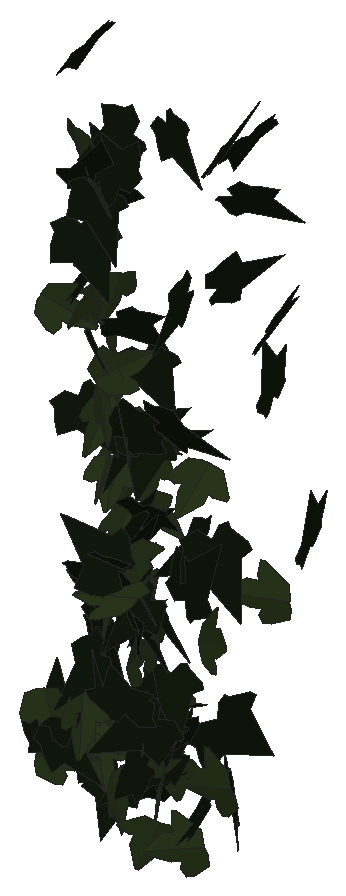
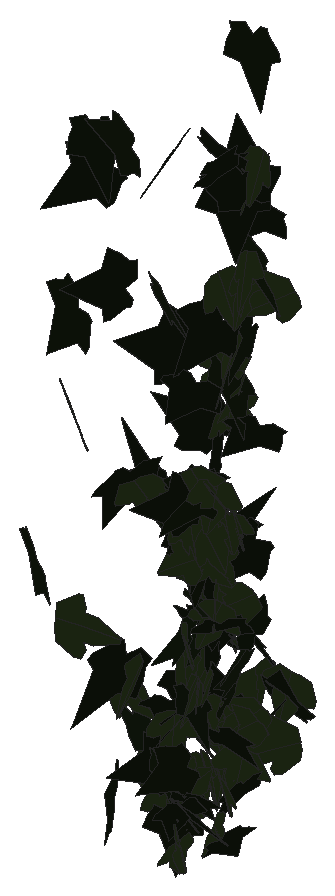
# SketchUp Ruby script. Lengths in inches.
U = 1.inch
M = Sketchup.active_model
def pt(a) = Geom::Point3d.new(a.map { |v| v * U })
def face(e, loops, mat)
  f = e.add_face(loops[0].map { |a| pt(a) })
  loops[1..].each { |l| e.add_face(l.map { |a| pt(a) }).erase! }
  f.material = f.back_material = mat if mat
  f
end
# faces: each face lists its corners as indices into pts; further lists are holes
def faces(e, pts, list, mat = nil) = list.each { |f| face(e, (f[0].is_a?(Array) ? f : [f]).map { |l| l.map { |i| pts[i] } }, mat) }
# xy, xz, yz: faces in a plane at the given z, y or x. An outline is a flat list of corners, or four numbers for a rectangle; further outlines are holes
def ring(l) = l.size == 4 ? [[l[0], l[1]], [l[2], l[1]], [l[2], l[3]], [l[0], l[3]]] : l.each_slice(2).to_a
def flat(e, list, mat, &to3) = list.each { |f| face(e, (f[0].is_a?(Array) ? f : [f]).map { |l| ring(l).map { |u, v| to3.(u, v) } }, mat) }
def xy(e, z, list, mat = nil) = flat(e, list, mat) { |x, y| [x, y, z] }
def xz(e, y, list, mat = nil) = flat(e, list, mat) { |x, z| [x, y, z] }
def yz(e, x, list, mat = nil) = flat(e, list, mat) { |y, z| [x, y, z] }
def lines(e, pts, list) = list.each { |a, b| e.add_line(pt(pts[a]), pt(pts[b])) }
# prism: a flat outline (further loops are holes) pulled along v
def prism(e, loops, v, mat = nil)
  f = face(e, loops, mat); d = Geom::Vector3d.new(v.map { |x| x * U })
  f.pushpull(f.normal.samedirection?(d) ? d.length : -d.length)
end
def box(e, o, s, mat = nil) = prism(e, [[o, [o[0] + s[0], o[1], o[2]], [o[0] + s[0], o[1] + s[1], o[2]], [o[0], o[1] + s[1], o[2]]]], [0, 0, s[2]], mat)
def at(x, y, z, deg = 0) = Geom::Transformation.translation(pt([x, y, z])) * Geom::Transformation.rotation(ORIGIN, Z_AXIS, deg.degrees)
def axes(o, x, y, z) = Geom::Transformation.new([*x, 0, *y, 0, *z, 0, *pt(o).to_a, 1])
def part(name) = M.definitions.add(name)
# library, detail: a bought-in or finely detailed component or shape, given as its bounding box
def library(name, o, s) = part(name).tap { |d| box(d.entities, o, s) }
def detail(e, o, s) = box(e.add_group.entities, o, s)
def put(e, d, t, mat = nil) = e.add_instance(d, t).tap { |i| i.material = mat if mat }
def group(e, t, mat = nil) = e.add_group.tap { |g| g.transformation = t; g.material = mat if mat }.entities
root = M.entities
M.materials.add("efeu1").color = [18, 25, 13]
M.materials.add("efeu2").color = [43, 57, 29]
c1 = part("ivyleaf_9")
p = [[1.54,2.16,1.25],[1.36,2.04,1.19],[-0.21,0.99,0.68],[-0.71,1.11,0.82],[-0.85,0.86,0.67],[-0.8,0.17,0.21],
  [-0.9,-0.01,0.1],[-0.67,-0.16,-0.02],[-0.08,-0.08,-0.05],[-0.03,-0.6,-0.4],[0.65,-0.88,-0.66],[0.83,-0.6,-0.49],
  [1.29,-0.42,-0.43],[1.8125,-0.07,-0.26],[1.21,0.44,0.15]]
faces(c1.entities,p,[[0,1,2,3,4,5,6,7,8,9,10,11,12,13,14]],"efeu1")
c2 = part("ivyleaf_10")
p = [[0,0.5,-0.03],[-0.0625,2.02,-0.43],[-0.19,2.01,-0.46],[-0.54,1.05,-0.29],[-0.52,0.625,-0.18],[-0.83,0.76,-0.28],
  [-1.16,0.64,-0.33],[-1.15,0.33,-0.24],[-0.77,-0.39,0.02],[-0.3,-0.51,0.16],[0.04,-0.48,0.23],[-0.02,2.01,-0.4375],
  [-0.06,2.01,-0.43],[0.04,-0.49,0.23],[0.67,-0.49,0.14],[1.38,0.36,-0.2],[1.375,0.51,-0.24],[0.81,0.65,-0.19],
  [0.62,0.59,-0.15],[0.6,1.09,-0.28],[0.5,1.23,-0.31]]
faces(c2.entities,p,[[0,1,2,3,4,5,6,7,8,9,10],[11,12,0,13,14,15,16,17,18,19,20]],"efeu2")
put(root,c1,axes([599.8,129.43,210.84],[-1.0094,0.32917,0.06825],[0.04265,-0.08885,1.05933],[0.33345,1.0078,0.0711]))
put(root,c2,axes([599.1875,129.7,212.04],[1.03048,0.1413,0.29449],[0.24667,0.30222,-1.00817],[-0.21411,1.02824,0.25585]))
put(root,c1,axes([600.84,130.04,234.19],[-0.38872,-0.56207,-0.84526],[0.63503,0.57147,-0.67204],[0.79191,-0.73416,0.12401]))
put(root,c1,axes([599.62,129.73,210.85],[0.65216,-0.64278,-0.53026],[-0.15877,0.56516,-0.88036],[0.81801,0.62216,0.25187]))
put(root,c2,axes([603.07,129.99,217.9375],[-0.04227,1.23527,0.10042],[-1.23885,-0.04494,0.03131],[0.03483,-0.09925,1.2356]))
put(root,c1,axes([603.22,129.6875,213.04],[-0.18269,1.18347,0.00538],[-1.18301,-0.18277,0.03272],[0.03315,-0.00033,1.19704]))
put(root,c2,axes([600.71,130.22,212.13],[0.2396,0.99661,-0.25674],[-0.03873,-0.25469,-1.02479],[-1.02842,0.24178,-0.02122]))
put(root,c1,axes([601.19,130.41,235.84],[0.22293,-1.02597,-0.19339],[0.03804,0.2056,-1.0469],[1.04335,0.21172,0.07949]))
put(root,c1,axes([606.04,130.19,219.01],[-0.46531,0.47847,0.92349],[0.59746,-0.70516,0.66638],[0.85135,0.75637,0.03708]))
put(root,c2,axes([599.44,129.83,230.4],[0.41584,0.19312,0.89669],[0.64054,0.64358,-0.43565],[-0.65656,0.75019,0.14291]))
put(root,c1,axes([601.23,130.51,214.45],[-1.01027,0.18239,-0.18284],[0.17994,-0.03243,-1.0266],[-0.18525,-1.02617,-0.00006]))
put(root,c1,axes([601.07,130.26,232.3],[-0.69225,0.82547,-0.08837],[0.06963,-0.05693,-1.07718],[-0.82726,-0.69554,-0.01671]))
put(root,c1,axes([601.88,130.83,218.54],[-0.42706,-1.03566,-0.02438],[0.04845,-0.04631,1.11851],[-1.03481,0.42524,0.06243]))
put(root,c1,axes([604.54,130.51,226.29],[0.76824,-0.32958,0.76916],[0.72035,-0.27086,-0.83555],[0.42582,1.05282,0.02582]))
put(root,c2,axes([599.08,130.1,209.22],[0.25287,-0.03046,1.00775],[0.47165,0.92184,-0.09049],[-0.89108,0.47929,0.23808]))
put(root,c2,axes([600.92,130.4375,230.94],[-0.13056,-0.88408,-0.57455],[0.04805,0.57335,-0.89315],[1.05328,-0.13575,-0.03047]))
put(root,c1,axes([600.72,130.33,242.4375],[-0.18071,1.07408,0.03515],[0.00614,0.03667,-1.08911],[-1.07464,-0.18041,-0.01214]))
put(root,c2,axes([600.95,130.64,235.82],[-0.88422,0.59693,0.11629],[-0.09585,0.06585,-1.06685],[-0.60055,-0.8894,-0.00094]))
put(root,c1,axes([600.37,131.18,235.6],[1.00501,0.36415,0.33832],[-0.31892,-0.11293,1.06895],[0.38125,-1.0544,0.00236]))
put(root,c1,axes([603.37,131.51,211.86],[-0.00613,-0.05087,-1.06175],[-0.40107,-0.98318,0.04942],[-0.9844,0.40089,-0.01352]))
put(root,c1,axes([600.66,130.45,218.5625],[0.94908,0.46168,0.16133],[0.12921,0.10297,-1.05482],[-0.47168,0.95718,0.03566]))
put(root,c2,axes([603.59,131.27,206.99],[-0.77742,-0.5951,0.43027],[-0.33296,-0.27283,-0.97896],[0.65453,-0.84562,0.01305]))
put(root,c1,axes([600.53,130.8125,228.82],[0.80974,-0.24262,-0.57743],[-0.55018,0.17548,-0.84527],[0.29931,0.97893,0.00841]))
put(root,c1,axes([602.11,130.7,236.35],[0.0561,0.38948,0.99667],[-0.74296,0.73244,-0.2444],[-0.7701,-0.67826,0.3084]))
put(root,c1,axes([601.125,130.84,235.37],[0.32356,0.9691,-0.29244],[-0.08667,-0.27937,-1.02167],[-1.00854,0.33492,-0.00602]))
put(root,c2,axes([605.35,131.48,206.74],[-0.33312,-0.03273,1.09339],[-1.00318,-0.44656,-0.31901],[0.43613,-1.05217,0.10138]))
put(root,c2,axes([600.78,131.63,225.24],[0.34032,0.79523,-0.57393],[-0.2388,-0.52202,-0.86491],[-0.95119,0.41557,0.0118]))
put(root,c2,axes([607.01,131.3125,210.14],[-0.38104,-0.01996,1.13302],[-1.13181,-0.05252,-0.38156],[0.05614,-1.19423,-0.00215]))
put(root,c2,axes([600.76,131.38,225.91],[-0.26255,0.99795,-0.1218],[0.00806,-0.12379,-1.03164],[-1.00532,-0.26162,0.02354]))
put(root,c2,axes([601.23,131.71,231.13],[-0.33562,-0.94792,0.23589],[-0.08153,-0.22137,-1.00558],[0.97343,-0.34537,-0.00289]))
put(root,c2,axes([599.59,131.36,237.41],[-0.91697,0.40198,0.01413],[-0.01262,0.00641,-1.00121],[-0.40203,-0.91706,-0.0008]))
put(root,c1,axes([605.89,131.68,208.81],[-0.81886,0.74891,-0.2525],[0.1762,-0.18144,-1.10959],[-0.77044,-0.83747,0.0146]))
put(root,c2,axes([601.17,131.21,227.05],[-0.2997,-0.43125,0.90814],[0.46576,0.78024,0.52423],[-0.89094,0.55296,-0.03143]))
put(root,c2,axes([601.32,131.5625,208.09],[-0.24681,0.99933,0.07458],[-0.11536,0.04796,-1.02446],[-0.99545,-0.25333,0.10023]))
put(root,c1,axes([601.14,131.31,226.83],[-0.30172,0.9805,0.14131],[-0.06821,0.1268,-1.0255],[-0.98828,-0.30809,0.02764]))
put(root,c1,axes([602.48,131.95,209.28],[-0.95299,0.34936,-0.02468],[0.01845,-0.02135,-1.01492],[-0.34975,-0.95307,0.01369]))
put(root,c1,axes([599.28,131.8,225.07],[-0.0914,-0.53308,-0.7751],[0.44979,0.6592,-0.50641],[0.82623,-0.41784,0.18994]))
put(root,c2,axes([602.02,132.51,211.35],[0.33567,-0.31147,0.88223],[0.68401,-0.5578,-0.45718],[0.63835,0.76149,0.02597]))
put(root,c1,axes([605.86,132.07,220.625],[0.10017,-1.00887,-0.62351],[-0.07039,0.61957,-1.0138],[1.18391,0.1222,-0.00752]))
put(root,c2,axes([599.81,132.28,209.26],[-0.93136,-0.34751,-0.17806],[0.27999,-0.27337,-0.93101],[0.27216,-0.90797,0.34846]))
put(root,c2,axes([599.78,131.91,232.73],[0.08944,-0.8559,-0.45372],[0.04234,0.45867,-0.85689],[0.9678,0.05903,0.07942]))
put(root,c1,axes([601.05,132.67,217.85],[-0.22222,0.11874,-0.90071],[0.72619,-0.53397,-0.24956],[-0.54592,-0.75864,0.03468]))
put(root,c1,axes([598.89,132.55,215.75],[0.2151,-0.43106,0.73589],[0.51536,-0.539,-0.46637],[0.67952,0.54524,0.12076]))
put(root,c2,axes([599.53,131.74,211.31],[0.42848,0.41091,0.72894],[0.42744,0.59656,-0.58754],[-0.71937,0.59922,0.08508]))
put(root,c2,axes([601.59,132.47,211.04],[-0.50006,-0.7858,0.31746],[-0.17079,-0.26761,-0.93142],[0.83012,-0.52842,-0.00039]))
put(root,c2,axes([599.62,131.95,210.86],[0.4762,0.36359,0.82375],[0.68136,0.46369,-0.59855],[-0.58865,0.83085,-0.02644]))
put(root,c1,axes([600.875,133.07,237.13],[-0.4316,-0.46592,0.7598],[-0.36677,-0.67656,-0.62322],[0.81231,-0.55303,0.12231]))
put(root,c1,axes([600.07,132.92,212.14],[0.02559,-0.4334,0.78524],[0.13379,-0.77493,-0.43206],[0.88687,0.12941,0.04253]))
put(root,c1,axes([601.66,132.05,224.06],[-0.01366,-0.03564,1.02045],[1.01916,-0.06295,0.01145],[0.0625,1.0186,0.03642]))
put(root,c2,axes([599.63,132.24,216.97],[-0.48048,-0.19059,-0.76031],[0.77591,0.01081,-0.49305],[0.11115,-0.89934,0.1552]))
put(root,c1,axes([601.31,131.82,229.36],[0.80399,0.59983,0.14538],[0.13325,0.06442,-1.00271],[-0.60264,0.81449,-0.02776]))
put(root,c1,axes([604.88,132.29,219.99],[-0.83526,0.69561,0.08091],[-0.06218,0.05178,-1.08698],[-0.69754,-0.83757,0]))
put(root,c2,axes([600.71,132.11,227.68],[-0.62054,0.6641,0.24978],[-0.14836,0.20304,-0.90843],[-0.69383,-0.63737,-0.02914]))
put(root,c2,axes([600.08,132.76,216],[0.63031,-0.60084,0.28748],[0.22448,-0.18102,-0.87051],[0.62711,0.66871,0.02266]))
put(root,c1,axes([600.52,133.0625,223.3],[-0.05924,-0.03696,0.93265],[0.17046,-0.91924,-0.0256],[0.91769,0.16836,0.06496]))
put(root,c1,axes([599.36,133.27,214.31],[0.05039,-0.69395,0.56336],[0.06187,-0.56019,-0.69558],[0.89169,0.07809,0.01643]))
put(root,c1,axes([600.74,133.15,214.24],[-0.08158,0.02672,0.92283],[0.37812,-0.84419,0.05787],[0.84223,0.38159,0.06341]))
put(root,c1,axes([601.73,133.17,216],[-0.92545,-0.2025,-0.0311],[0.04224,-0.04781,-0.94571],[0.20047,-0.92474,0.0557]))
put(root,c1,axes([599.26,132.8,208.46],[0.28296,-0.70848,-0.43848],[-0.0731,0.44019,-0.7584],[0.82998,0.2803,0.0827]))
put(root,c1,axes([599.25,133.08,214],[0.50809,-0.71757,0.10254],[0.06783,-0.0776,-0.87918],[0.72167,0.5125,0.01045]))
put(root,c1,axes([603.57,133.17,230.7],[-0.83899,0.30198,-0.47884],[0.44223,-0.18486,-0.89143],[-0.35343,-0.94816,0.0213]))
put(root,c1,axes([601.45,133.19,219.93],[-0.75783,0.5106,-0.30044],[0.17456,-0.27372,-0.90548],[-0.56614,-0.76789,0.12299]))
put(root,c2,axes([599.44,133.21,221.57],[0.63829,-0.65031,0.05837],[0.04512,-0.03751,-0.91119],[0.65136,0.63985,0.00592]))
put(root,c1,axes([599.92,133.39,210.93],[-0.84292,-0.22041,-0.05985],[0.05668,0.01981,-0.87124],[0.22125,-0.84481,-0.00482]))
put(root,c2,axes([601.27,132.71,218.11],[0.25652,0.89548,0.30349],[-0.19345,0.35752,-0.89137],[-0.92551,0.17347,0.27044]))
put(root,c1,axes([600.96,133.27,215.18],[0.64562,-0.68494,0.10224],[0.06737,-0.077,-0.94125],[0.68924,0.64912,-0.00377]))
put(root,c2,axes([601.45,132.5,213.3125],[-0.0015,0.02926,0.97798],[-0.56843,0.79597,-0.02468],[-0.79635,-0.56821,0.01578]))
put(root,c2,axes([600.54,132.78,217.3],[0.1416,-0.59992,-0.71314],[-0.17055,0.69246,-0.61639],[0.91618,0.22163,-0.00452]))
put(root,c2,axes([600.23,133.48,219.13],[0.38012,0.6937,-0.42512],[-0.27017,-0.33498,-0.78818],[-0.76743,0.46152,0.06691]))
put(root,c2,axes([599.59,133.41,221.28],[0.88662,0.2075,0.01562],[0.01413,0.00815,-0.91056],[-0.20761,0.88672,0.00471]))
put(root,c1,axes([605.75,132.65,212.17],[0.08057,-0.26114,-1.21709],[-0.41394,1.14461,-0.27299],[1.17395,0.42151,-0.01273]))
put(root,c1,axes([601.83,134.03,211.48],[-0.21072,-0.84422,0.28513],[-0.07493,-0.27517,-0.8701],[0.88792,-0.22357,-0.00576]))
put(root,c1,axes([600.375,133.85,222.92],[-0.75671,-0.05778,-0.5191],[0.51333,-0.25092,-0.72037],[-0.09639,-0.88267,0.23876]))
put(root,c1,axes([601.39,133.36,227.03],[-0.31266,-0.41689,-0.80022],[0.46293,0.65284,-0.52098],[0.7745,-0.5585,-0.01166]))
put(root,c1,axes([601.14,133.67,217.18],[-0.75616,0.44442,-0.0887],[-0.00275,-0.17705,-0.8636],[-0.45318,-0.74047,0.15325]))
put(root,c1,axes([601.86,134.06,210.89],[0.10719,-0.91126,0.18831],[0.01773,-0.18752,-0.91753],[0.93034,0.10856,-0.00421]))
put(root,c1,axes([601.07,133.99,222.98],[-0.43297,-0.79055,-0.16017],[0.14116,0.10471,-0.89844],[0.79417,-0.44961,0.07238]))
put(root,c1,axes([601.53,133.11,219.28],[-0.03773,0.94926,0.08622],[0.00821,0.08661,-0.94993],[-0.95313,-0.03683,-0.0116]))
put(root,c1,axes([601.35,133.27,220.13],[0.63342,0.47937,-0.53501],[-0.52366,-0.18016,-0.78139],[-0.49175,0.80932,0.14295]))
put(root,c1,axes([602.39,133.55,237.86],[0.59549,-0.71626,-0.37598],[-0.21134,0.3129,-0.93082],[0.78085,0.63092,0.03479]))
put(root,c1,axes([599.28,134.14,206.43],[-0.24984,-0.80875,0.07936],[-0.02589,-0.07506,-0.84646],[0.81222,-0.25117,-0.00258]))
put(root,c1,axes([599.59,133.9,216.47],[-0.30243,-0.73216,-0.38905],[0.24412,0.31714,-0.78658],[0.79235,-0.37716,0.09384]))
put(root,c2,axes([601.54,133.77,213.92],[0.10082,-0.91383,-0.15298],[0.01167,0.15512,-0.91894],[0.92647,0.0975,0.02822]))
put(root,c2,axes([599.33,134.04,209.02],[0.69543,-0.46742,0.16983],[0.13493,-0.10366,-0.83785],[0.47866,0.70832,-0.01054]))
put(root,c2,axes([599.9375,133.72,216.84],[-0.72314,-0.38845,-0.33887],[0.33546,0.08864,-0.81747],[0.39139,-0.79367,0.07455]))
put(root,c2,axes([600.48,133.78,209.62],[0.5791,-0.55595,-0.37786],[-0.24547,0.2894,-0.802],[0.62578,0.628,0.03508]))
put(root,c2,axes([599.68,134.1875,206.8],[-0.05778,0.64432,-0.51881],[-0.03335,-0.52147,-0.6439],[-0.82656,-0.024,0.06225]))
put(root,c1,axes([601.32,133.9,215.38],[0.73112,-0.59081,-0.03105],[-0.00884,0.03844,-0.93968],[0.59156,0.73077,0.02432]))
put(root,c2,axes([599.95,134.24,220.59],[-0.12845,-0.8267,0.34846],[-0.02397,-0.34873,-0.83616],[0.89682,-0.12772,0.02756]))
put(root,c2,axes([601.51,134.28,207.52],[0.55395,-0.57966,0.44731],[0.3316,-0.30146,-0.80132],[0.65278,0.64503,0.02747]))
put(root,c1,axes([604.9375,133.33,237.11],[-0.37057,0.98119,-0.11102],[-0.04073,0.1033,1.04884],[0.98661,0.3728,0.00159]))
put(root,c1,axes([601.95,134.29,212.15],[-0.31912,-0.70797,-0.46638],[0.35826,0.33903,-0.75979],[0.76836,-0.45212,0.16056]))
put(root,c2,axes([600.59,134.33,223.22],[-0.735,-0.21801,0.51141],[-0.38015,-0.42148,-0.72603],[0.40564,-0.79001,0.24622]))
put(root,c1,axes([605.95,133.55,235.88],[0.94453,0.39886,0.3907],[0.34913,0.17725,-1.02497],[-0.43572,1.00666,0.02567]))
put(root,c2,axes([599.72,134.1,222.87],[-0.8552,-0.32834,-0.08377],[0.07615,0.03539,-0.91604],[0.33019,-0.85856,-0.00572]))
put(root,c2,axes([603.4375,134.43,221.89],[0.77132,0.47593,-0.43617],[-0.36803,-0.23416,-0.90631],[-0.53038,0.8546,-0.00543]))
put(root,c2,axes([601.08,134.04,208.24],[-0.61148,0.31904,-0.65953],[-0.57892,0.3161,0.68965],[0.44902,0.842,-0.009]))
put(root,c2,axes([601.76,134.35,211.26],[-0.77206,-0.46864,-0.01357],[0.01109,0.00789,-0.90316],[0.46871,-0.77214,-0.00099]))
put(root,c2,axes([600.69,134.57,221.27],[-0.53161,-0.72343,0.14926],[0.03389,-0.20759,-0.88543],[0.73789,-0.51166,0.1482]))
put(root,c2,axes([599.94,134.28,213.73],[-0.47082,0.72127,0.07951],[-0.05801,0.05707,-0.86116],[-0.72332,-0.47406,0.0173]))
put(root,c2,axes([600.66,134.87,215.81],[0.5848,-0.57903,0.30021],[0.23604,-0.18799,-0.8224],[0.60801,0.6299,0.03052]))
put(root,c1,axes([600.48,134.01,222.66],[0.77672,0.47728,0.09717],[-0.02959,0.22879,-0.8873],[-0.48618,0.74859,0.20924]))
put(root,c1,axes([602.03,134.8,208.35],[-0.8357,0.30864,-0.11911],[0.10291,-0.06502,-0.89052],[-0.31441,-0.84164,0.02512]))
put(root,c2,axes([601.88,134.63,207.84],[-0.70012,-0.52973,-0.02388],[0.01862,0.01498,-0.87794],[0.52994,-0.70037,-0.00071]))
put(root,c2,axes([600.69,134.64,219.4],[0.46509,0.0199,0.76704],[0.73454,0.24774,-0.45181],[-0.22181,0.86214,0.11213]))
put(root,c1,axes([605.76,134.54,238.16],[-0.18166,1.02509,-0.18651],[0.02221,-0.18547,-1.04101],[-1.04169,-0.18272,0.01033]))
put(root,c1,axes([601.51,134.43,206.98],[0.1472,0.89947,-0.04674],[-0.14715,-0.02271,-0.90041],[-0.88859,0.15276,0.14137]))
put(root,c1,axes([604.5,134.26,230.94],[0.28576,0.23677,0.96316],[0.72306,0.63636,-0.37096],[-0.6789,0.77741,0.01032]))
put(root,c1,axes([602.02,134.57,209.12],[-0.34214,0.77698,0.33054],[-0.11698,0.30959,-0.84881],[-0.83622,-0.36121,-0.0165]))
put(root,c1,axes([601.84,134.47,209.35],[0.62752,0.2369,0.62073],[0.54682,0.30082,-0.66761],[-0.37738,0.82981,0.06481]))
put(root,c1,axes([603.81,135.72,207.49],[0.14309,-0.02543,-1.18926],[1.13618,-0.35177,0.14423],[-0.35224,-1.14502,-0.0179]))
put(root,c1,axes([600.71,134.59,222],[0.32485,0.2365,0.81663],[0.68246,0.4488,-0.40145],[-0.50701,0.75564,-0.01715]))
put(root,c1,axes([599.89,135.73,208.96],[-0.69698,-0.39305,-0.15288],[0.20019,-0.04842,-0.78817],[0.37119,-0.7119,0.13801]))
put(root,c2,axes([599.76,135.37,214],[-0.62824,0.60557,-0.01651],[-0.07835,-0.10481,-0.86287],[-0.60071,-0.61965,0.12982]))
put(root,c1,axes([599.99,135.34,213.5625],[-0.35218,0.79212,-0.04949],[0.01499,-0.04749,-0.86686],[-0.79352,-0.35245,0.00559]))
put(root,c1,axes([606.55,134.75,229.4],[0.12589,0.78452,0.91321],[0.09506,0.90885,-0.79387],[-1.20016,0.15428,0.03291]))
put(root,c1,axes([600.51,135.15,209.87],[0.6225,0.37429,0.41969],[0.22731,0.40518,-0.6985],[-0.51436,0.63205,0.19924]))
put(root,c1,axes([599.95,135.93,208.42],[-0.76302,0.22794,0.16029],[-0.17478,-0.02753,-0.79281],[-0.21704,-0.77919,0.0749]))
put(root,c2,axes([599.65,135.46,214.07],[0.20589,-0.55728,-0.63968],[0.05859,0.66601,-0.56137],[0.84635,0.08946,0.19447]))
put(root,c1,axes([599.93,136.13,208.67],[-0.10505,-0.74354,-0.37416],[0.05646,0.36989,-0.75091],[0.83045,-0.1192,0.00372]))
put(root,c2,axes([602.98,135.31,213.61],[-0.27998,0.48729,0.89992],[-0.43648,0.78702,-0.56195],[-0.92563,-0.51851,-0.00722]))
put(root,c2,axes([605.35,136.83,215.79],[-0.05918,-0.05426,1.16376],[-1.04423,-0.51422,-0.07708],[0.51659,-1.04566,-0.02248]))
put(root,c2,axes([599.6,136.65,207.11],[0.11692,0.77451,-0.16715],[-0.02454,-0.16534,-0.78328],[-0.79196,0.11946,-0.00041]))
put(root,c2,axes([599.32,136.82,206.5],[0.38063,-0.65917,-0.25275],[0.13165,-0.21583,0.76115],[-0.69358,-0.40271,0.00577]))
put(root,c1,axes([605.55,136.27,225.53],[-0.12871,0.41681,1.05418],[-0.35743,0.99191,-0.43583],[-1.07576,-0.37944,0.01868]))
put(root,c1,axes([606.57,137.4,218.55],[-0.13317,0.55146,1.06771],[-0.23023,1.04264,-0.56723],[-1.17945,-0.26579,-0.00983]))
